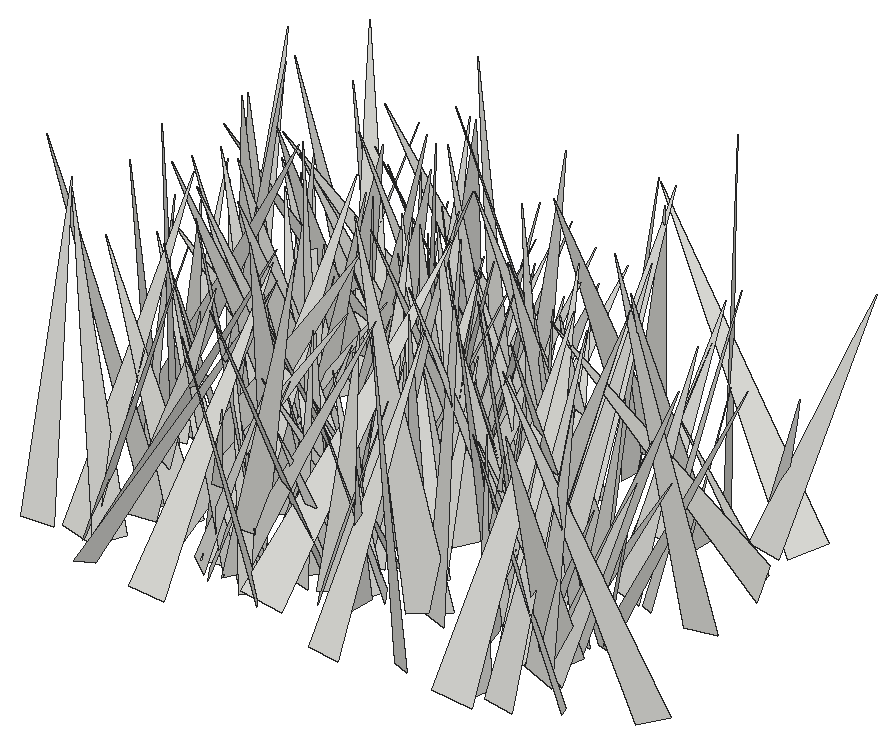
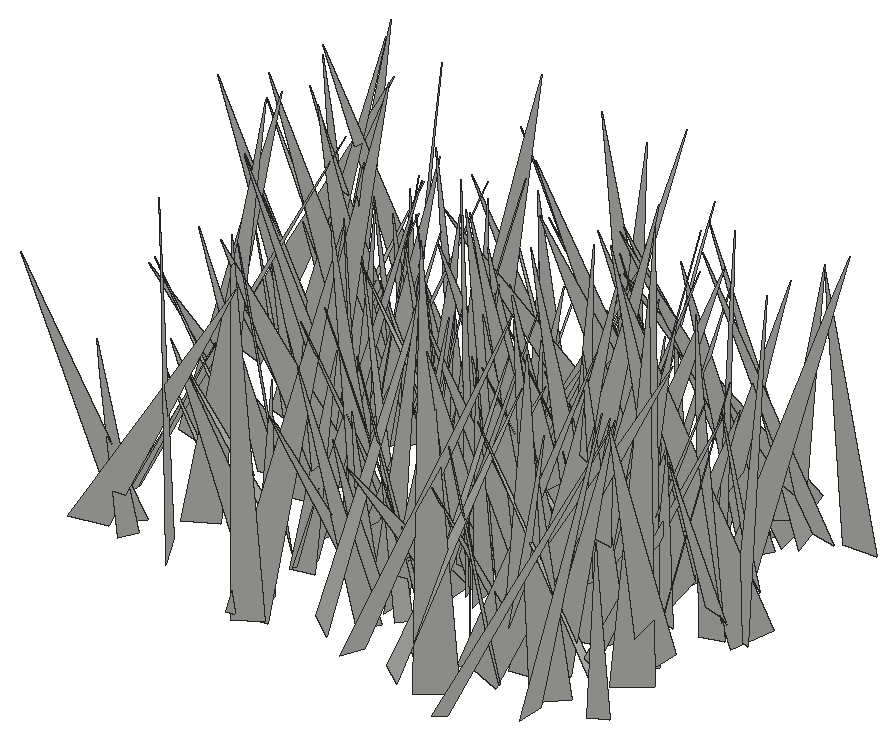
# SketchUp Ruby script. Lengths in inches.
U = 1.inch
M = Sketchup.active_model
def pt(a) = Geom::Point3d.new(a.map { |v| v * U })
def face(e, loops, mat)
  f = e.add_face(loops[0].map { |a| pt(a) })
  loops[1..].each { |l| e.add_face(l.map { |a| pt(a) }).erase! }
  f.material = f.back_material = mat if mat
  f
end
# faces: each face lists its corners as indices into pts; further lists are holes
def faces(e, pts, list, mat = nil) = list.each { |f| face(e, (f[0].is_a?(Array) ? f : [f]).map { |l| l.map { |i| pts[i] } }, mat) }
# xy, xz, yz: faces in a plane at the given z, y or x. An outline is a flat list of corners, or four numbers for a rectangle; further outlines are holes
def ring(l) = l.size == 4 ? [[l[0], l[1]], [l[2], l[1]], [l[2], l[3]], [l[0], l[3]]] : l.each_slice(2).to_a
def flat(e, list, mat, &to3) = list.each { |f| face(e, (f[0].is_a?(Array) ? f : [f]).map { |l| ring(l).map { |u, v| to3.(u, v) } }, mat) }
def xy(e, z, list, mat = nil) = flat(e, list, mat) { |x, y| [x, y, z] }
def xz(e, y, list, mat = nil) = flat(e, list, mat) { |x, z| [x, y, z] }
def yz(e, x, list, mat = nil) = flat(e, list, mat) { |y, z| [x, y, z] }
def lines(e, pts, list) = list.each { |a, b| e.add_line(pt(pts[a]), pt(pts[b])) }
# prism: a flat outline (further loops are holes) pulled along v
def prism(e, loops, v, mat = nil)
  f = face(e, loops, mat); d = Geom::Vector3d.new(v.map { |x| x * U })
  f.pushpull(f.normal.samedirection?(d) ? d.length : -d.length)
end
def box(e, o, s, mat = nil) = prism(e, [[o, [o[0] + s[0], o[1], o[2]], [o[0] + s[0], o[1] + s[1], o[2]], [o[0], o[1] + s[1], o[2]]]], [0, 0, s[2]], mat)
def at(x, y, z, deg = 0) = Geom::Transformation.translation(pt([x, y, z])) * Geom::Transformation.rotation(ORIGIN, Z_AXIS, deg.degrees)
def axes(o, x, y, z) = Geom::Transformation.new([*x, 0, *y, 0, *z, 0, *pt(o).to_a, 1])
def part(name) = M.definitions.add(name)
# library, detail: a bought-in or finely detailed component or shape, given as its bounding box
def library(name, o, s) = part(name).tap { |d| box(d.entities, o, s) }
def detail(e, o, s) = box(e.add_group.entities, o, s)
def put(e, d, t, mat = nil) = e.add_instance(d, t).tap { |i| i.material = mat if mat }
def group(e, t, mat = nil) = e.add_group.tap { |g| g.transformation = t; g.material = mat if mat }.entities
root = M.entities
c1 = part("fur_instance\#9")
p = [[0.8125,0,1.79],[0.67,-0.02,1.48],[0,-0.11,0],[0,0.11,0]]
faces(c1.entities,p,[[0,1,2,3]])
put(root,c1,axes([87.53,443.96,-27.1],[-6.45449,2.84921,1.13675],[2.42101,6.35763,-2.18855],[1.88385,1.59157,6.70736]))
put(root,c1,axes([86.75,448.39,-27.1],[-1.48065,3.15767,1.46809],[3.42197,1.61497,-0.02236],[0.64523,-1.31889,3.48751]))
put(root,c1,axes([87.33,440.55,-27.1],[0.66443,5.27954,0.01832],[5.19176,-0.65673,0.9642],[-0.95891,0.10252,5.2331]))
put(root,c1,axes([86.32,440.66,-27.1],[-2.86307,-5.78602,1.82095],[-5.78172,3.21211,1.11581],[1.83453,1.09334,6.35847]))
put(root,c1,axes([87.1,432.75,-27.1],[-0.4945,6.57851,1.5324],[6.75453,0.47319,0.14829],[-0.03697,-1.53911,6.5954]))
put(root,c1,axes([89.69,436.38,-27.1],[-2.64388,-6.79077,2.11498],[-6.99476,2.07362,-2.08599],[-1.28885,2.67645,6.98236]))
put(root,c1,axes([88.76,436.82,-27.1],[2.37609,4.94692,0.8109],[4.47755,-2.49789,2.11838],[-2.25414,0.25283,5.06264]))
put(root,c1,axes([88.87,449.6875,-27.1],[-6.26748,-0.84521,1.62615],[-0.68504,6.45447,0.7145],[1.69984,-0.51518,6.28372]))
put(root,c1,axes([87.25,445.78,-27.1],[5.45655,-4.97036,1.37233],[-4.9464,-5.60993,-0.6508],[-1.45634,0.43117,7.35221]))
put(root,c1,axes([89.48,441.29,-27.1],[-0.14147,5.00237,0.6936],[4.87308,-0.04695,1.33257],[-1.32587,-0.70632,4.82369]))
put(root,c1,axes([89.54,445.4,-27.1],[-5.28354,-0.86585,0.73138],[-0.45173,4.80676,2.42722],[1.0395,-2.31209,4.77222]))
put(root,c1,axes([87.22,441.21,-27.1],[-0.17668,-5.97479,1.5156],[-5.97573,0.53792,1.42395],[1.51188,1.4279,5.80532]))
put(root,c1,axes([90.06,433.28,-27.1],[-6.40273,2.01611,1.14645],[1.98655,6.50456,-0.34415],[1.19695,-0.01086,6.70383]))
put(root,c1,axes([90.98,442,-27.1],[-5.83458,-0.97839,0.23219],[-1.00024,5.78729,-0.74851],[0.10327,0.77686,5.8685]))
put(root,c1,axes([88.99,438.46,-27.1],[-4.49865,-5.44108,2.87885],[-5.83326,4.90701,0.15896],[1.96626,2.10876,7.05818]))
put(root,c1,axes([90.92,438.45,-27.1],[-2.13288,4.47426,0.69403],[4.36785,1.83113,1.61826],[-1.19274,-1.2953,4.68502]))
put(root,c1,axes([87.81,444.65,-27.1],[7.83218,-2.47016,1.5817],[-2.12062,-7.88445,-1.81244],[-2.02643,-1.29626,8.00998]))
put(root,c1,axes([89.88,440.57,-27.1],[-3.92886,-2.51502,0.86647],[-2.44083,4.02285,0.60923],[1.05758,-0.05874,4.62495]))
put(root,c1,axes([89.96,446.86,-27.1],[3.58153,-3.37168,2.12142],[-3.21603,-4.13077,-1.13573],[-2.3507,0.51427,4.78599]))
put(root,c1,axes([88.83,432.88,-27.1],[1.55056,7.17303,0.47228],[7.18686,-1.53634,-0.26142],[0.15632,-0.51668,7.33405]))
put(root,c1,axes([86,440.35,-27.1],[7.56022,-3.29271,0.03526],[-3.23696,-7.41517,1.59297],[0.60437,1.47429,8.09082]))
put(root,c1,axes([91.37,451.83,-27.1],[-6.30471,-1.37126,0.42808],[-1.05468,5.72683,2.8114],[0.97532,-2.67133,5.80738]))
put(root,c1,axes([92.08,448.55,-27.1],[-0.45254,-7.13046,0.09555],[-6.72101,0.39447,-2.39372],[-2.38342,0.24148,6.7319]))
put(root,c1,axes([91.16,443.02,-27.1],[-3.95377,2.90545,0.68572],[2.92437,3.99824,-0.07937],[0.59996,-0.34142,4.90588]))
put(root,c1,axes([91.32,441.49,-27.1],[-4.7653,3.97573,1.88545],[4.327,4.73874,0.94381],[0.79899,-1.95123,6.13381]))
put(root,c1,axes([91.64,435.82,-27.1],[-5.50696,2.25656,1.40845],[2.52369,5.45565,1.12666],[0.84072,-1.59571,5.84374]))
put(root,c1,axes([90.08,439.4,-27.1],[-7.4216,0.05563,3.73189],[-0.80703,8.0859,-1.72548],[3.64401,1.90407,7.21845]))
put(root,c1,axes([92.2,446.68,-27.1],[-6.19983,-0.76734,1.02255],[-1.02443,6.01091,-1.70052],[0.76483,1.83095,6.01123]))
put(root,c1,axes([89.79,443.79,-27.1],[5.47744,-1.647,1.93505],[-1.81976,-5.75174,0.25556],[-1.77356,0.81501,5.71398]))
put(root,c1,axes([89.24,445.81,-27.1],[4.55508,3.875,0.43107],[3.83788,-4.57312,0.55448],[-0.68713,0.14532,5.95457]))
put(root,c1,axes([91.88,442.53,-27.1],[0.79588,-7.21699,0.96951],[-7.03929,-1.01213,-1.75565],[-1.86367,0.74092,7.04528]))
put(root,c1,axes([91.71,446.49,-27.1],[-3.76745,6.43232,1.47995],[6.58457,3.78058,0.33053],[0.45645,-1.44608,7.44709]))
put(root,c1,axes([91.01,444.4,-27.1],[4.14575,-5.15062,1.64406],[-4.88287,-4.45639,-1.64839],[-2.32151,0.17524,6.40304]))
put(root,c1,axes([89.0625,433.39,-27.1],[6.34041,1.92452,0.88463],[1.94009,-6.39712,0.01179],[-0.84995,-0.24555,6.62604]))
put(root,c1,axes([90.61,447.52,-27.1],[1.9178,-7.47283,0.23219],[-7.45531,-1.92947,-0.52008],[-0.56157,0.09505,7.69744]))
put(root,c1,axes([88.92,448.45,-27.1],[3.49272,-6.19271,0.17705],[-6.11252,-3.41157,1.25629],[1.00898,0.76914,6.99789]))
put(root,c1,axes([90.65,443.27,-27.1],[2.6007,2.51832,0.88377],[2.64819,-2.58836,-0.41733],[-0.33183,-0.9193,3.59603]))
put(root,c1,axes([92.97,441.51,-27.1],[0.07199,5.81915,0.58708],[5.58747,-0.24194,1.7129],[-1.72841,-0.53974,5.5618]))
put(root,c1,axes([89.8,435.3125,-27.1],[3.48254,-4.50934,1.30252],[-4.66936,-3.1635,1.53235],[0.47726,1.95368,5.48763]))
put(root,c1,axes([92.88,448.3,-27.1],[-6.34287,-0.8603,1.40577],[-0.30586,6.10717,2.3574],[1.61949,-2.21602,5.95103]))
put(root,c1,axes([93.32,442.15,-27.1],[-6.61379,-2.13915,0.88077],[-1.88588,6.53057,1.69974],[1.33985,-1.36736,6.74011]))
put(root,c1,axes([89.66,433.34,-27.1],[7.04502,0.38941,0.11832],[0.34745,-6.82295,1.76766],[-0.21195,1.75889,6.83077]))
put(root,c1,axes([91.37,448.49,-27.1],[3.19088,3.17646,1.19509],[3.39239,-3.03309,-0.99593],[-0.09903,-1.55252,4.39087]))
put(root,c1,axes([90.33,431.46,-27.1],[6.45135,0.1489,0.38361],[-0.04006,-5.77049,2.9136],[-0.40954,2.91007,5.75787]))
put(root,c1,axes([90.03,437.41,-27.1],[5.30447,3.34271,0.68413],[3.37643,-4.96043,-1.94241],[0.49141,-1.99988,5.96139]))
put(root,c1,axes([93.6,440.27,-27.1],[-4.4668,1.24969,0.75909],[0.98308,4.37301,-1.41442],[1.08236,1.18546,4.4174]))
put(root,c1,axes([94.96,434.33,-27.1],[-6.17227,-0.98801,0.5453],[-1.07692,6.06305,-1.2042],[0.3373,1.27815,6.13375]))
put(root,c1,axes([91.24,446.69,-27.1],[1.22352,3.80068,0.33063],[3.61313,-1.04295,-1.38167],[1.22465,-0.72012,3.74608]))
put(root,c1,axes([94.63,450.55,-27.1],[-3.64802,-5.0358,0.07825],[-5.03596,3.64854,0.02575],[0.06676,0.04827,6.21825]))
put(root,c1,axes([93.2,442.625,-27.1],[6.13444,-4.45258,1.42838],[-3.84619,-6.14459,-2.6359],[-2.65943,-1.38408,7.10696]))
put(root,c1,axes([94.9,439.7,-27.1],[-3.18645,2.79123,0.05753],[2.78151,3.16651,0.42911],[-0.23972,-0.36053,4.21429]))
put(root,c1,axes([94.1,446.6875,-27.1],[2.37526,2.53476,1.46683],[2.25858,-2.78775,1.16004],[-1.86424,-0.14786,3.27432]))
put(root,c1,axes([94.6,442.51,-27.1],[-4.83197,-1.5354,1.95575],[-2.0901,4.8234,-1.3772],[1.34681,1.9768,4.87942]))
put(root,c1,axes([90.8,440.84,-27.1],[4.14208,3.82367,0.06036],[3.46383,-3.71363,-2.44781],[1.62049,-1.8356,5.07794]))
put(root,c1,axes([92.94,435.68,-27.1],[3.65052,-1.24636,0.3015],[-1.17659,-3.61738,-0.70767],[-0.50984,-0.576,3.79195]))
put(root,c1,axes([94.84,449.02,-27.1],[-4.07639,-4.57708,0.71562],[-4.52519,4.13816,0.69067],[0.99219,0.06853,6.09012]))
put(root,c1,axes([96.16,434.875,-27.1],[-6.23091,-2.8217,1.23434],[-3.03851,6.08694,-1.42355],[0.50305,1.81577,6.69027]))
put(root,c1,axes([95.55,447.58,-27.1],[-6.52757,-2.25287,1.08541],[-2.07972,6.57544,1.14066],[1.38863,-0.74224,6.81054]))
put(root,c1,axes([92.75,441.23,-27.1],[6.6153,-1.38256,1.33275],[-1.44359,-6.733,0.18083],[-1.26639,0.45296,6.75581]))
put(root,c1,axes([93.57,431.02,-27.1],[-1.05391,6.67902,0.37292],[6.52998,1.10912,-1.41007],[1.4518,-0.14015,6.613]))
put(root,c1,axes([90.14,437.95,-27.1],[3.5795,-7.50714,1.0436],[-6.77337,-2.6505,4.166],[3.40115,2.62237,7.19823]))
put(root,c1,axes([96.78,450.14,-27.1],[-7.42366,-0.80204,0.92134],[-0.52005,7.2098,2.08597],[1.1053,-1.9946,7.16957]))
put(root,c1,axes([95.62,443.98,-27.1],[-5.53054,0.45224,1.5037],[0.10523,5.59989,-1.29715],[1.5667,1.22031,5.39525]))
put(root,c1,axes([93.49,439.15,-27.1],[6.57894,-4.30915,0.69378],[-4.10201,-6.53322,-1.6802],[-1.49116,-1.03963,7.68298]))
put(root,c1,axes([96.48,433.36,-27.1],[-4.58917,0.765,0.19448],[0.68534,4.43094,-1.25723],[0.3916,1.21042,4.47941]))
put(root,c1,axes([92.49,450.63,-27.1],[2.66865,-7.95792,0.14871],[-7.80747,-2.5868,1.68053],[1.54726,0.67254,8.22351]))
put(root,c1,axes([93.77,433.84,-27.1],[2.51167,3.62255,0.80621],[3.69421,-2.34748,-0.96099],[0.35452,-1.20325,4.30208]))
put(root,c1,axes([91.45,435.46,-27.1],[4.41498,5.25807,0.18984],[4.81628,-3.93899,-2.90917],[2.11822,-2.00311,6.21901]))
put(root,c1,axes([94.46,434.4,-27.1],[-4.73234,6.09922,1.47861],[5.53404,4.92888,-2.61961],[2.95993,0.53615,7.26177]))
put(root,c1,axes([93.85,438.77,-27.1],[3.11489,-2.67244,0.85057],[-2.80172,-2.90834,1.1224],[0.12545,1.40269,3.94774]))
put(root,c1,axes([97.53,436.11,-27.1],[-7.91635,-0.39433,1.24518],[-0.80795,7.48837,-2.76517],[1.02625,2.85367,7.42819]))
put(root,c1,axes([94.41,437.8125,-27.1],[3.13129,2.44329,0.37399],[2.42945,-3.15346,0.26073],[-0.45532,-0.0231,3.96316]))
put(root,c1,axes([93.42,443.15,-27.1],[6.3266,0.04535,0.7535],[-0.10627,-6.24313,1.26797],[-0.74735,1.27161,6.1984]))
put(root,c1,axes([95.32,439.09,-27.1],[3.44077,4.42208,0.21812],[4.18127,-3.33634,1.68138],[-1.45578,0.8691,5.34478]))
put(root,c1,axes([94.44,433.54,-27.1],[3.52648,2.43175,0.31475],[2.41999,-3.54045,0.23962],[-0.3951,0.0194,4.27692]))
put(root,c1,axes([94.0625,441.9,-27.1],[7.6269,-0.50277,1.8471],[-0.68475,-7.80192,0.70374],[-1.78765,0.84341,7.61099]))
put(root,c1,axes([95.7,438.93,-27.1],[-1.12897,-3.54048,0.33773],[-3.515,1.16474,0.46018],[0.54205,0.17891,3.68752]))
put(root,c1,axes([93.47,444.38,-27.1],[6.15872,-4.73604,0.69713],[-4.78091,-6.14284,0.50431],[-0.2428,0.82545,7.75278]))
put(root,c1,axes([97.04,442.55,-27.1],[-6.53703,2.92768,0.70077],[2.53956,6.26275,-2.47462],[1.61648,2.00045,6.72163]))
put(root,c1,axes([97.3,438.88,-27.1],[-3.1283,2.85302,0.75954],[2.94685,2.94951,1.058],[-0.18092,-1.28978,4.09959]))
put(root,c1,axes([95.36,441.16,-27.1],[2.13777,3.57515,0.4757],[3.58502,-2.16686,0.17428],[-0.39447,-0.3179,4.1619]))
put(root,c1,axes([96.4,440.97,-27.1],[-5.56085,2.56326,1.5764],[2.25423,5.74256,-1.38556],[1.99343,0.65656,5.96435]))
put(root,c1,axes([96.88,433.34,-27.1],[-4.48858,-3.56813,1.07524],[-3.58767,4.5928,0.2643],[1.00813,0.45789,5.72792]))
put(root,c1,axes([98.68,442.05,-27.1],[-3.99392,-3.16377,0.39905],[-3.06383,3.62986,-1.88605],[-0.88412,1.71311,4.73326]))
put(root,c1,axes([97.68,446.46,-27.1],[-6.3571,-0.05635,1.63328],[-0.03082,6.56286,0.10646],[1.63396,-0.09544,6.35645]))
put(root,c1,axes([96.58,442.88,-27.1],[-2.91269,3.59929,0.76549],[3.33369,2.99435,-1.39463],[1.55801,0.3218,4.41516]))
put(root,c1,axes([98.8125,445.58,-27.1],[1.70019,7.5386,2.42367],[7.33263,-2.43467,2.42902],[-2.9895,-1.68439,7.33628]))
put(root,c1,axes([96.32,441.91,-27.1],[-1.6675,3.7386,1.84502],[3.94069,2.06209,-0.61692],[1.36097,-1.39013,4.04687]))
put(root,c1,axes([96.51,444.43,-27.1],[-3.43381,3.18637,0.41007],[2.54254,3.06224,-2.50406],[1.96382,1.60682,3.959]))
put(root,c1,axes([95.36,434.4,-27.1],[6.75458,-3.1446,1.55563],[-3.25939,-6.87331,0.25842],[-1.29802,0.89549,7.44621]))
put(root,c1,axes([99.4,438.24,-27.1],[-2.79932,-5.24784,0.26282],[-5.09915,2.64134,-1.57068],[-1.26789,0.96362,5.73663]))
put(root,c1,axes([97.47,435.03,-27.1],[1.36793,4.62634,1.5435],[4.80198,-1.5578,0.41343],[-0.85231,-1.35162,4.8066]))
put(root,c1,axes([96.35,443.72,-27.1],[7.03768,2.72348,2.80411],[3.28727,-7.24831,-1.21043],[-2.11523,-2.20318,7.44856]))
put(root,c1,axes([98.35,438.68,-27.1],[-4.30266,-2.43803,0.04686],[-2.30354,4.09498,1.544],[0.79994,-1.32144,4.69819]))
put(root,c1,axes([96.23,446.68,-27.1],[3.37327,4.28522,1.21914],[4.44713,-3.33099,-0.5966],[-0.2692,-1.33033,5.4209]))
put(root,c1,axes([97.9375,436.02,-27.1],[-3.38776,-6.42257,0.32475],[-6.36234,3.40084,0.88702],[0.93573,-0.12917,7.20691]))
put(root,c1,axes([95.72,439.125,-27.1],[2.4486,-4.30122,0.69777],[-4.269,-2.2075,1.37318],[0.8735,1.26866,4.75506]))
put(root,c1,axes([97.27,443.57,-27.1],[3.86717,-5.0611,1.49434],[-5.13106,-4.03908,-0.40116],[-1.23289,0.93486,6.35679]))
put(root,c1,axes([99.17,439.25,-27.1],[-0.33006,-3.76044,0.39687],[-3.50265,0.15395,-1.45434],[-1.42474,0.49269,3.4835]))
put(root,c1,axes([98.72,443.93,-27.1],[3.89411,3.28531,3.07479],[3.51498,-4.75969,0.63397],[-2.80935,-1.40135,5.05524]))
put(root,c1,axes([98.88,449.33,-27.1],[-4.98525,-6.36904,1.05647],[-6.36247,5.07321,0.56124],[1.09531,0.48105,8.06861]))
put(root,c1,axes([98.56,436.3,-27.1],[0.67909,-3.62862,0.46379],[-3.53581,-0.77205,-0.86319],[-0.93808,0.2832,3.58928]))
put(root,c1,axes([99.17,441.47,-27.1],[-0.52973,-5.32119,2.08202],[-5.65742,0.19488,-0.94137],[-0.8022,2.1395,5.26399]))
put(root,c1,axes([98.46,445.84,-27.1],[-3.60567,-4.25836,0.82426],[-4.10665,3.69659,1.13335],[1.39586,-0.12438,5.46351]))
put(root,c1,axes([98.67,437.45,-27.1],[-5.11212,3.73872,1.49873],[3.53116,5.32488,-1.23875],[1.93782,0.15985,6.21106]))
put(root,c1,axes([98,438.05,-27.1],[3.54062,0.10617,1.20258],[0.38468,-3.63127,-0.812],[-1.14433,-0.89222,3.44788]))
put(root,c1,axes([95.1,434.31,-27.1],[5.1253,5.35023,0.94765],[5.22805,-4.50107,-2.86349],[1.48003,-2.62814,6.83331]))
put(root,c1,axes([101.08,438.22,-27.1],[-1.83761,6.5724,0.07775],[6.30696,1.74042,1.94227],[-1.85059,-0.59481,6.54223]))
put(root,c1,axes([98.95,444.22,-27.1],[-6.12859,-4.53414,1.24355],[-3.97845,6.08997,2.59781],[2.50535,-1.42065,7.16724]))
put(root,c1,axes([97.22,433.16,-27.1],[-2.37553,7.32496,0.20013],[6.77476,2.27563,-2.87444],[2.79244,0.71043,7.14393]))
put(root,c1,axes([98.68,437.24,-27.1],[6.48387,0.57283,2.72889],[-0.5216,-6.53637,2.61139],[-2.73914,2.60063,5.96233]))
put(root,c1,axes([98.31,446.8,-27.1],[-2.24113,2.46388,1.48853],[2.36542,2.65133,-0.82724],[1.6405,-0.45695,3.22631]))
put(root,c1,axes([96.9375,445.74,-27.1],[4.58071,3.98416,0.78034],[4.05613,-4.44078,-1.1369],[0.17387,-1.36793,5.96354]))
put(root,c1,axes([96.59,441.56,-27.1],[5.74165,3.30721,0.02247],[3.30582,-5.73764,-0.2359],[0.09829,-0.21562,6.62182]))
put(root,c1,axes([100.63,445.15,-27.1],[-4.67838,0.58429,0.4377],[0.60816,4.68963,0.24018],[0.40387,-0.29353,4.7086]))
put(root,c1,axes([96.875,443.55,-27.1],[6.48852,0.93317,0.66882],[1.0636,-6.33108,-1.48501],[-0.43231,-1.57025,6.38486]))
put(root,c1,axes([100.11,436.02,-27.1],[-4.10178,1.61092,0.95507],[1.70987,4.15942,0.32775],[0.76391,-0.66031,4.39457]))
put(root,c1,axes([96.75,447.1875,-27.1],[6.70588,0.95076,0.50826],[1.07552,-6.12086,-2.74035],[-0.07444,-2.78609,6.19381]))
put(root,c1,axes([99.87,445.37,-27.1],[-4.04138,0.55951,1.25439],[0.25517,4.13619,-1.02282],[1.34961,0.89343,3.94964]))
put(root,c1,axes([98.82,435.4,-27.1],[3.55242,-4.27149,1.91187],[-4.60398,-3.6203,0.46613],[-0.83917,1.77997,5.53606]))
put(root,c1,axes([100.48,436.32,-27.1],[-3.61255,-2.36918,0.54232],[-2.35627,3.65218,0.25916],[0.59592,0.07847,4.31235]))
put(root,c1,axes([97.49,448.3,-27.1],[1.64693,-4.65446,0.85777],[-4.4282,-1.19483,2.01879],[1.67056,1.42146,4.50564]))
put(root,c1,axes([100.48,441.34,-27.1],[-5.43342,3.18473,2.47254],[3.60205,5.6984,0.57576],[1.81141,-1.77869,6.27161]))
put(root,c1,axes([98.97,446.36,-27.1],[-0.26739,4.57604,0.32256],[4.40279,0.34673,-1.26925],[1.2883,-0.2352,4.40462]))
put(root,c1,axes([98.54,441.8,-27.1],[5.36268,3.16176,1.79895],[3.56295,-5.21159,-1.4615],[-0.73371,-2.1986,6.05138]))
put(root,c1,axes([98.375,444.19,-27.1],[2.55836,5.15566,0.46861],[5.11042,-2.43162,-1.14739],[0.82709,-0.92305,5.63999]))
put(root,c1,axes([98.47,434.97,-27.1],[4.57096,2.53062,0.74602],[2.63797,-4.36083,-1.37058],[0.04077,-1.55993,5.04174]))
put(root,c1,axes([99.73,445.26,-27.1],[6.98669,-0.82296,2.45735],[-1.02769,-7.36659,0.45485],[-2.37901,0.76535,7.02027]))
put(root,c1,axes([99.84,439.11,-27.1],[-1.49561,-5.63035,1.67127],[-5.71638,1.79132,0.91926],[1.34798,1.34949,5.75262]))
put(root,c1,axes([99.83,439.9,-27.1],[4.69636,2.95892,0.9191],[2.85112,-4.78039,0.82137],[-1.21287,0.21986,5.48965]))
put(root,c1,axes([100.23,435.21,-27.1],[3.94789,-1.4658,0.35037],[-1.34081,-3.86465,-1.06014],[-0.68816,-0.87925,4.0756]))
put(root,c1,axes([102.52,436.32,-27.1],[2.49125,-7.31611,3.2771],[-7.62751,-3.2193,-1.38865],[-2.46697,2.5655,7.60286]))
put(root,c1,axes([102.23,446.1,-27.1],[-7.41474,-1.37074,2.09218],[-0.74138,7.45582,2.25736],[2.38883,-1.94072,7.19456]))
put(root,c1,axes([101.4,450.52,-27.1],[2.31085,-7.14722,0.11909],[-7.10013,-2.30949,-0.83147],[-0.82765,-0.14321,7.46535]))
put(root,c1,axes([101.95,446.63,-27.1],[1.41164,-4.04262,0.99191],[-4.10193,-1.52908,-0.39425],[-0.70768,0.79907,4.26381]))
put(root,c1,axes([101.4,431.5,-27.1],[0.40052,6.46259,0.29319],[6.45769,-0.38185,-0.40475],[0.38629,-0.31712,6.46233]))
put(root,c1,axes([102.47,442.96,-27.1],[-6.58404,0.20466,2.39247],[0.20033,7.00521,-0.04793],[2.39284,-0.02336,6.58705]))
put(root,c1,axes([102.81,443.92,-27.1],[-3.06168,2.49465,0.02952],[2.42804,2.99025,-0.87237],[0.57338,0.65813,3.85176]))
put(root,c1,axes([102,437.03,-27.1],[-0.34341,4.80516,0.97397],[4.88667,0.41477,-0.32328],[0.39826,-0.94579,4.80656]))
put(root,c1,axes([103.02,436,-27.1],[2.9733,6.47594,2.08154],[6.51847,-3.36189,1.14821],[-1.94427,-1.36785,7.03277]))
put(root,c1,axes([101.875,448.92,-27.1],[3.65469,-1.69105,0.3912],[-1.57801,-3.61693,-0.89287],[-0.72291,-0.65395,3.92673]))
put(root,c1,axes([104.22,432.51,-27.1],[-3.8782,-4.63911,2.52217],[-5.26639,3.62608,-1.42825],[0.38461,2.87286,5.87554]))
put(root,c1,axes([101.23,450.68,-27.1],[0.69431,-7.1025,1.01226],[-6.95299,-0.41552,1.85354],[1.7681,1.15502,6.89145]))
put(root,c1,axes([105.63,438.77,-27.1],[-6.50715,-2.26194,0.29712],[-2.26712,6.51165,-0.07913],[0.25462,0.17236,6.88863]))
put(root,c1,axes([103.8,445.09,-27.1],[4.42049,5.15695,1.86392],[5.12768,-4.73588,0.94203],[-1.94301,-0.76574,6.72662]))
put(root,c1,axes([103.47,441.39,-27.1],[-3.24328,-4.06122,2.56752],[-4.33534,3.80899,0.54855],[2.07134,1.61325,5.16831]))
put(root,c1,axes([105.125,438.75,-27.1],[-5.04486,-3.51647,1.75014],[-3.733,5.17856,-0.35556],[1.22196,1.30239,6.1392]))
put(root,c1,axes([105.37,438.31,-27.1],[4.87258,-2.82126,2.84071],[-2.53321,-5.63755,-1.25383],[-3.10033,0.17232,5.48903]))
put(root,c1,axes([104.79,440.72,-27.1],[-5.35866,5.61511,0.59327],[5.12673,5.1813,-2.73266],[2.36603,1.4904,7.2648]))
put(root,c1,axes([104.35,437.86,-27.1],[-6.11732,-3.75265,2.76683],[-3.28898,6.70851,1.82699],[3.3046,-0.26993,6.94018]))
put(root,c1,axes([105.375,442.48,-27.1],[3.52334,-7.25518,1.10129],[-7.15699,-3.66725,-1.26216],[-1.62106,0.42196,7.96608]))
put(root,c1,axes([107.02,435.63,-27.1],[0.33091,4.05955,1.18914],[3.81261,-0.80293,1.68011],[-1.83248,-0.93747,3.71034]))
put(root,c1,axes([104.64,436.6,-27.1],[4.0424,-1.6774,0.68877],[-1.67315,-4.09915,-0.16314],[-0.69903,0.11126,4.37357]))
put(root,c1,axes([105.11,445.875,-27.1],[-1.9043,4.31856,1.08738],[4.14528,2.15112,-1.28374],[1.62757,-0.42591,4.54184]))
put(root,c1,axes([105.32,444.21,-27.1],[3.38702,2.66566,0.2184],[2.51461,-3.29384,1.20529],[-0.91115,0.81867,4.13823]))
put(root,c1,axes([105.49,436.36,-27.1],[4.4988,1.24272,1.44893],[1.33102,-4.70119,-0.10058],[-1.36826,-0.48722,4.6662]))
put(root,c1,axes([106.66,448.45,-27.1],[6.19858,3.66698,3.16063],[3.75526,-6.8827,0.6206],[-3.05522,-1.01998,7.17523]))
put(root,c1,axes([108.26,437.99,-27.1],[1.91991,5.69676,2.84026],[5.7974,-2.78995,1.67703],[-2.62873,-1.9923,5.77292]))
put(root,c1,axes([110.4,448.5,-27.1],[-5.51381,4.9525,0.02994],[4.6746,5.18943,2.47955],[-1.63592,-1.86355,6.98435]))
put(root,c1,axes([106.25,441.04,-27.1],[4.13039,-0.87619,1.21239],[-0.99071,-4.26996,0.28929],[-1.12075,0.54542,4.21238]))
put(root,c1,axes([106.25,438.44,-27.1],[1.83288,7.01444,0.75411],[7.05484,-1.82448,-0.17632],[-0.01908,-0.77421,7.24781]))
put(root,c1,axes([107.74,432.9,-27.1],[-4.70779,-0.34884,1.44292],[-0.70643,4.74641,-1.15738],[1.30563,1.3103,4.57662]))
put(root,c1,axes([108.62,437.18,-27.1],[-4.68733,-0.90911,0.30449],[-0.85582,4.65242,0.7161],[0.43216,-0.64711,4.72067]))
put(root,c1,axes([107.44,435.37,-27.1],[-5.06165,5.7028,1.49455],[5.55918,5.27278,-1.292],[1.96243,-0.22764,7.51486]))
put(root,c1,axes([105.26,437.32,-27.1],[6.69732,-3.52244,1.21858],[-3.71872,-6.48437,1.69431],[-0.25228,2.07171,7.37503]))
put(root,c1,axes([108.17,443.71,-27.1],[2.52886,2.74781,0.4271],[2.47453,-2.48701,1.34889],[-1.2687,0.62635,3.48225]))
put(root,c1,axes([107.13,446.03,-27.1],[6.98894,-3.62557,1.01436],[-3.15649,-6.80873,-2.58782],[-2.05189,-1.87497,7.43594]))
put(root,c1,axes([107.12,431.84,-27.1],[-0.59068,7.87895,1.19707],[7.83923,0.79048,-1.33468],[1.43434,-1.07565,7.78752]))
put(root,c1,axes([107.39,441.7,-27.1],[0.7475,5.23214,1.319],[5.34274,-0.53135,-0.92008],[0.75507,-1.41992,5.20456]))
put(root,c1,axes([107.23,435.45,-27.1],[6.03648,4.13261,1.07509],[4.02235,-6.12795,0.97074],[-1.43354,0.20766,7.25088]))
put(root,c1,axes([110.875,433.66,-27.1],[-4.67684,-2.75,0.36196],[-2.71074,4.38122,-1.73872],[-0.58771,1.67594,5.13928]))
put(root,c1,axes([108.48,441.48,-27.1],[3.77258,4.9169,0.38845],[4.64704,-3.70729,1.79444],[-1.65279,0.7995,5.93196]))
put(root,c1,axes([110.65,445.57,-27.1],[-7.29463,-2.71144,0.02018],[-2.47986,6.69465,3.09773],[1.09665,-2.89718,7.13916]))
put(root,c1,axes([107.1875,438.99,-27.1],[3.6219,-1.04912,0.12415],[-1.02885,-3.40219,1.26523],[0.23987,1.24847,3.55218]))
put(root,c1,axes([108.77,432.5,-27.1],[1.7832,7.11152,0.69499],[7.11724,-1.83129,0.47737],[-0.63379,-0.55606,7.31612]))
put(root,c1,axes([109.58,438.125,-27.1],[-2.16653,-7.31637,0.90738],[-7.36569,2.18851,0.05952],[0.3151,0.85299,7.63018]))
put(root,c1,axes([107.79,435.77,-27.1],[3.74369,-0.67268,0.40161],[-0.71907,-3.7286,0.45768],[-0.31101,0.52348,3.776]))
put(root,c1,axes([110.54,445.73,-27.1],[-3.53813,-0.73541,0.01575],[-0.72603,3.50386,0.50526],[0.11809,-0.49152,3.57826]))
put(root,c1,axes([108.72,438.87,-27.1],[3.70099,1.78589,1.07617],[1.91017,-3.78303,-0.29128],[-0.83593,-0.7377,4.09901]))
put(root,c1,axes([111.08,441.41,-27.1],[-1.04276,-7.37455,2.60053],[-7.71345,0.53914,-1.56404],[-1.28435,2.74945,7.28184]))
put(root,c1,axes([108.3,440.05,-27.1],[5.03908,0.51167,0.65236],[0.18588,-4.61324,2.18248],[-0.80798,2.12978,4.57066]))
put(root,c1,axes([108.6,448.41,-27.1],[3.31097,-1.72543,0.32906],[-1.73993,-3.31791,0.10944],[-0.24091,0.24944,3.73197]))
put(root,c1,axes([108.84,436.23,-27.1],[5.9537,-4.05045,0.58701],[-3.75603,-5.81897,-2.05648],[-1.62572,-1.38951,6.90098]))
put(root,c1,axes([108.59,435.08,-27.1],[1.5633,5.69815,3.01797],[6.40687,-1.02237,-1.38843],[0.72737,-3.24142,5.74326]))
put(root,c1,axes([109.0625,435.42,-27.1],[2.45412,4.72767,0.6627],[4.74881,-2.3413,-0.8831],[0.48874,-0.99004,5.25297]))
put(root,c1,axes([108.24,437.07,-27.1],[6.2285,-2.9564,0.62521],[-3.02175,-6.08711,1.31964],[0.01382,1.46019,6.76705]))
put(root,c1,axes([113.85,435.15,-27.1],[-2.36054,6.29762,2.85628],[6.53149,1.03928,3.10644],[-2.27111,-3.55673,5.96508]))
put(root,c1,axes([109.125,447.5,-27.1],[-0.64371,5.67181,1.6895],[5.48083,1.21245,-1.9821],[2.23257,-1.34117,5.35305]))
